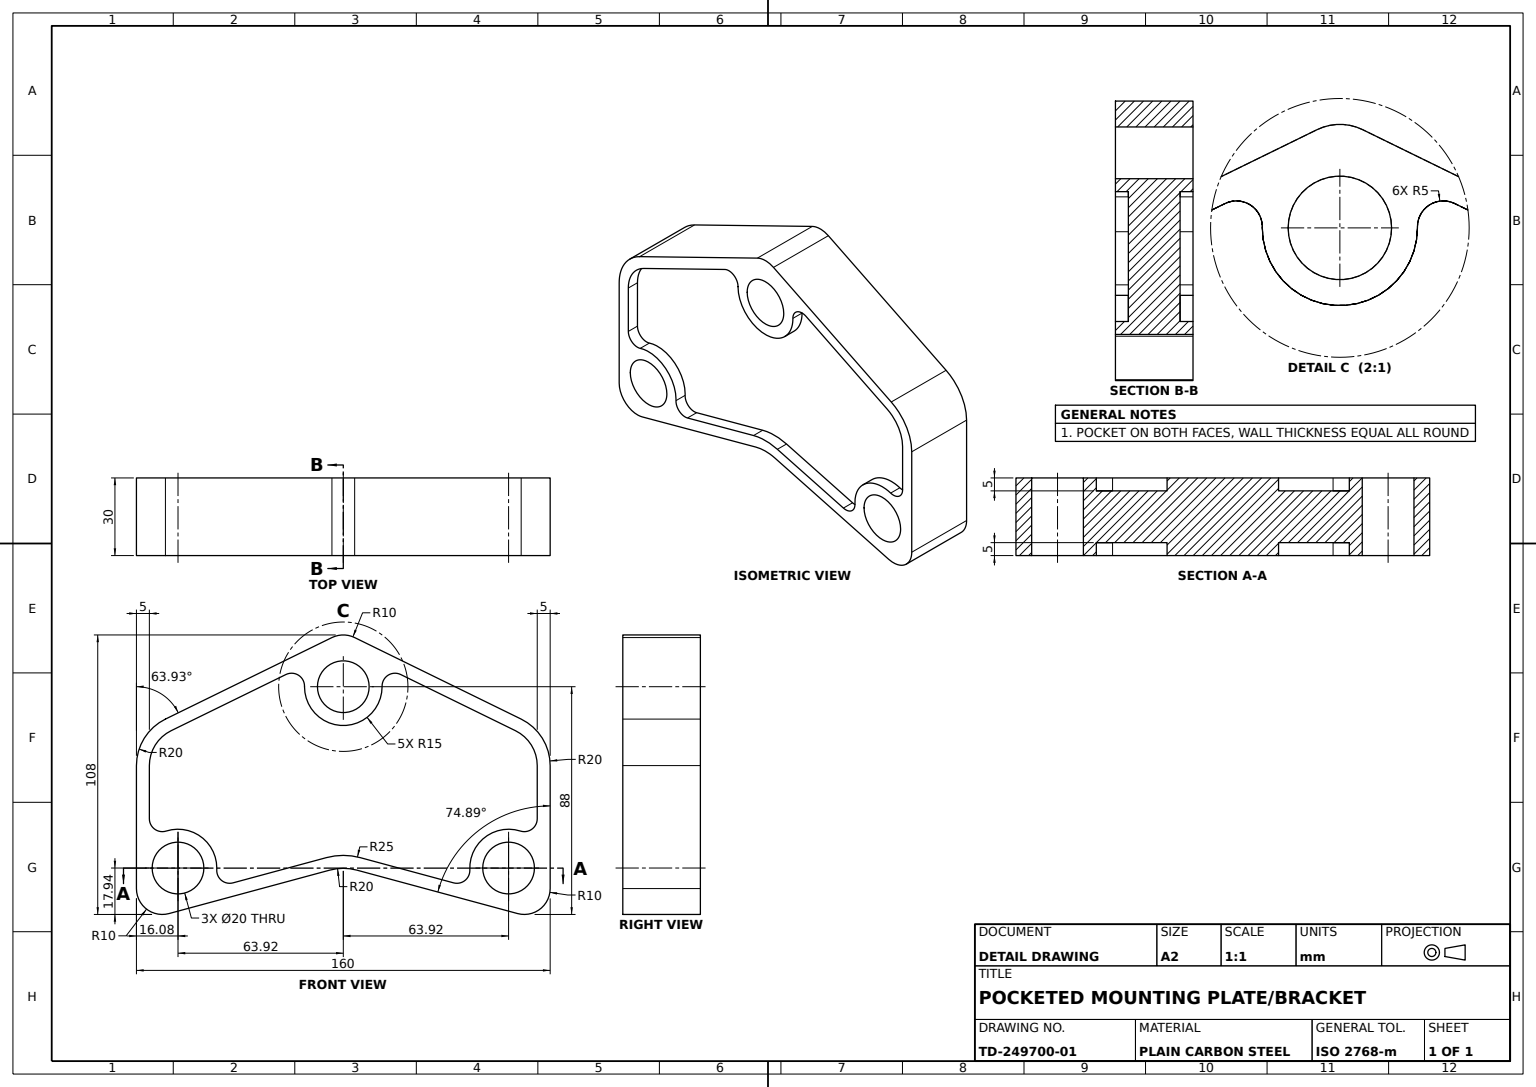
solid
v1 (-15,-10,15)
v2 (15,-10,15)
e1 v1 v2 CIRCLE(AX(P(0,-10,15),D(0,0,1),D(1,0,0)),15)
v3 (-15,-10,10)
e2 v3 v1 LINE
v4 (15,-10,10)
e3 v3 v4 CIRCLE(AX(P(0,-10,10),D(0,0,1),D(1,0,0)),15)
e4 v4 v2 LINE
face CYL(AX(P(0,-10,10),D(0,0,1),D(1,0,0)),15) [-e1 -e2 e3 e4]
v5 (-80,-40.481445,15)
v6 (-80,-88,15)
e5 v5 v6 LINE
v7 (-80,-40.481445,-15)
e6 v5 v7 LINE
v8 (-80,-88,-15)
e7 v7 v8 LINE
e8 v6 v8 LINE
face PLANE(AX(P(-80,-88,15),D(1,0,0),D(0,0,-1))) rev [-e5 e6 e7 -e8]
v9 (75,-61.007005,-15)
v10 (75,-40.481445,-15)
e9 v9 v10 LINE
v11 (75,-61.007005,-10)
e10 v11 v9 LINE
v12 (75,-40.481445,-10)
e11 v11 v12 LINE
e12 v12 v10 LINE
face PLANE(AX(P(75,-61.007005,-10),D(-1,0,0),D(0,-1,0))) [-e9 -e10 e11 e12]
v13 (-14.999113,-9.836864,-10)
v14 (-22.195826,-5.291032,-10)
e13 v13 v14 CIRCLE(AX(P(-19.998817,-9.782485,-10),D(0,0,1),D(1,0,0)),5)
v15 (-22.195826,-5.291032,-15)
e14 v14 v15 LINE
v16 (-14.999113,-9.836864,-15)
e15 v16 v15 CIRCLE(AX(P(-19.998817,-9.782485,-15),D(0,0,1),D(1,0,0)),5)
e16 v13 v16 LINE
face CYL(AX(P(-19.998817,-9.782485,-10),D(0,0,-1),D(-1,0,0)),5) rev [e13 e14 -e15 -e16]
v17 (-48.935435,-80.737052,10)
v18 (-42.636957,-85.789651,10)
e17 v17 v18 CIRCLE(AX(P(-43.940523,-80.96257,10),D(0,0,1),D(1,0,0)),5)
v19 (-48.935435,-80.737052,15)
e18 v17 v19 LINE
v20 (-42.636957,-85.789651,15)
e19 v19 v20 CIRCLE(AX(P(-43.940523,-80.96257,15),D(0,0,1),D(1,0,0)),5)
e20 v18 v20 LINE
face CYL(AX(P(-43.940523,-80.96257,10),D(0,0,1),D(1,0,0)),5) rev [-e17 e18 e19 -e20]
v21 (-15,-10,-10)
v22 (-15,-10,-15)
e21 v21 v22 LINE
e22 v13 v21 CIRCLE(AX(P(0,-10,-10),D(0,0,1),D(1,0,0)),15)
e23 v16 v22 CIRCLE(AX(P(0,-10,-15),D(0,0,1),D(1,0,0)),15)
face CYL(AX(P(0,-10,-10),D(0,0,-1),D(-1,0,0)),15) [-e21 -e22 e16 e23]
v23 (-4.394017,8.982907,15)
v24 (-4.394017,8.982907,-15)
e24 v23 v24 LINE
v25 (4.394017,8.982907,15)
e25 v25 v23 CIRCLE(AX(P(0,0,15),D(0,0,1),D(1,0,0)),10)
v26 (4.394017,8.982907,-15)
e26 v25 v26 LINE
e27 v26 v24 CIRCLE(AX(P(0,0,-15),D(0,0,1),D(1,0,0)),10)
face CYL(AX(P(0,0,15),D(0,0,-1),D(-1,0,0)),10) [-e24 -e25 e26 e27]
v27 (-48.920169,-80.0605,10)
v28 (-48.920169,-80.0605,15)
e28 v27 v28 LINE
v29 (-68.480042,-65.770379,10)
e29 v27 v29 CIRCLE(AX(P(-63.920169,-80.0605,10),D(0,0,1),D(1,0,0)),15)
v30 (-68.480042,-65.770379,15)
e30 v29 v30 LINE
e31 v28 v30 CIRCLE(AX(P(-63.920169,-80.0605,15),D(0,0,1),D(1,0,0)),15)
face CYL(AX(P(-63.920169,-80.0605,10),D(0,0,1),D(1,0,0)),15) [-e28 e29 e30 -e31]
v31 (-75,-40.481445,-10)
v32 (-75,-61.007005,-10)
e32 v31 v32 LINE
v33 (-75,-61.007005,-15)
e33 v32 v33 LINE
v34 (-75,-40.481445,-15)
e34 v34 v33 LINE
e35 v31 v34 LINE
face PLANE(AX(P(-75,-40.481445,-10),D(1,0,0),D(0,0,-1))) [e32 e33 -e34 -e35]
v35 (-75,-61.007005,15)
e36 v35 v30 CIRCLE(AX(P(-70,-61.007005,15),D(0,0,1),D(1,0,0)),5)
v36 (-75,-61.007005,10)
e37 v36 v29 CIRCLE(AX(P(-70,-61.007005,10),D(0,0,1),D(1,0,0)),5)
e38 v36 v35 LINE
face CYL(AX(P(-70,-61.007005,10),D(0,0,1),D(1,0,0)),5) rev [e36 -e30 -e37 e38]
v37 (48.935435,-80.737052,-10)
v38 (48.920169,-80.0605,-10)
e39 v37 v38 CIRCLE(AX(P(63.920169,-80.0605,-10),D(0,0,-1),D(-1,0,0)),15)
v39 (42.636957,-85.789651,-10)
e40 v37 v39 CIRCLE(AX(P(43.940523,-80.96257,-10),D(0,0,-1),D(-1,0,0)),5)
v40 (6.51783,-76.035586,-10)
e41 v40 v39 LINE
v41 (-6.51783,-76.035586,-10)
e42 v40 v41 CIRCLE(AX(P(0,-100.170994,-10),D(0,0,1),D(1,0,0)),25)
v42 (-42.636957,-85.789651,-10)
e43 v42 v41 LINE
v43 (-48.940523,-80.96257,-10)
e44 v43 v42 CIRCLE(AX(P(-43.940523,-80.96257,-10),D(0,0,1),D(1,0,0)),5)
v44 (-48.935435,-80.737052,-10)
e45 v44 v43 CIRCLE(AX(P(-43.940523,-80.96257,-10),D(0,0,1),D(1,0,0)),5)
v45 (-68.480042,-65.770379,-10)
e46 v44 v45 CIRCLE(AX(P(-63.920169,-80.0605,-10),D(0,0,1),D(1,0,0)),15)
e47 v32 v45 CIRCLE(AX(P(-70,-61.007005,-10),D(0,0,1),D(1,0,0)),5)
v46 (-66.591026,-27.007085,-10)
e48 v46 v31 CIRCLE(AX(P(-60,-40.481445,-10),D(0,0,1),D(1,0,0)),15)
e49 v14 v46 LINE
v47 (15,-10,-10)
e50 v21 v47 CIRCLE(AX(P(0,-10,-10),D(0,0,1),D(1,0,0)),15)
v48 (14.999113,-9.836864,-10)
e51 v47 v48 CIRCLE(AX(P(0,-10,-10),D(0,0,1),D(1,0,0)),15)
v49 (14.998817,-9.782485,-10)
e52 v48 v49 CIRCLE(AX(P(19.998817,-9.782485,-10),D(0,0,-1),D(-1,0,0)),5)
v50 (22.195826,-5.291032,-10)
e53 v49 v50 CIRCLE(AX(P(19.998817,-9.782485,-10),D(0,0,-1),D(-1,0,0)),5)
v51 (66.591026,-27.007085,-10)
e54 v51 v50 LINE
e55 v12 v51 CIRCLE(AX(P(60,-40.481445,-10),D(0,0,1),D(1,0,0)),15)
v52 (68.480042,-65.770379,-10)
e56 v11 v52 CIRCLE(AX(P(70,-61.007005,-10),D(0,0,-1),D(-1,0,0)),5)
e57 v38 v52 CIRCLE(AX(P(63.920169,-80.0605,-10),D(0,0,-1),D(-1,0,0)),15)
face PLANE(AX(P(70,-61.007005,-10),D(0,0,1),D(-1,0,0))) rev [-e39 e40 -e41 e42 -e43 -e44 -e45 e46 -e47 -e32 -e48 -e49 -e13 e22 e50 e51 e52 e53 -e54 -e55 -e11 e56 -e57]
v53 (14.998817,-9.782485,-15)
e58 v49 v53 LINE
v54 (22.195826,-5.291032,-15)
e59 v53 v54 CIRCLE(AX(P(19.998817,-9.782485,-15),D(0,0,-1),D(-1,0,0)),5)
e60 v50 v54 LINE
face CYL(AX(P(19.998817,-9.782485,-10),D(0,0,-1),D(-1,0,0)),5) rev [e58 e59 -e60 -e53]
v55 (42.636957,-85.789651,10)
v56 (42.636957,-85.789651,15)
e61 v55 v56 LINE
v57 (6.51783,-76.035586,10)
e62 v57 v55 LINE
v58 (6.51783,-76.035586,15)
e63 v57 v58 LINE
e64 v58 v56 LINE
face PLANE(AX(P(6.51783,-76.035586,10),D(-0.260713207,-0.965416296,0),D(0.965416296,-0.260713207,0))) rev [-e61 -e62 e63 e64]
v59 (-53.920169,-80.0605,15)
v60 (-73.920169,-80.0605,15)
e65 v59 v60 CIRCLE(AX(P(-63.920169,-80.0605,15),D(0,0,1),D(1,0,0)),10)
e66 v60 v59 CIRCLE(AX(P(-63.920169,-80.0605,15),D(0,0,1),D(1,0,0)),10)
v61 (-14.998817,-9.782485,15)
v62 (-22.195826,-5.291032,15)
e67 v61 v62 CIRCLE(AX(P(-19.998817,-9.782485,15),D(0,0,1),D(1,0,0)),5)
v63 (-14.999113,-9.836864,15)
e68 v63 v61 CIRCLE(AX(P(-19.998817,-9.782485,15),D(0,0,1),D(1,0,0)),5)
e69 v63 v1 CIRCLE(AX(P(0,-10,15),D(0,0,1),D(1,0,0)),15)
v64 (14.999113,-9.836864,15)
e70 v2 v64 CIRCLE(AX(P(0,-10,15),D(0,0,1),D(1,0,0)),15)
v65 (22.195826,-5.291032,15)
e71 v64 v65 CIRCLE(AX(P(19.998817,-9.782485,15),D(0,0,-1),D(-1,0,0)),5)
v66 (66.591026,-27.007085,15)
e72 v66 v65 LINE
v67 (75,-40.481445,15)
e73 v67 v66 CIRCLE(AX(P(60,-40.481445,15),D(0,0,1),D(1,0,0)),15)
v68 (75,-61.007005,15)
e74 v68 v67 LINE
v69 (68.480042,-65.770379,15)
e75 v68 v69 CIRCLE(AX(P(70,-61.007005,15),D(0,0,-1),D(-1,0,0)),5)
v70 (48.935435,-80.737052,15)
e76 v70 v69 CIRCLE(AX(P(63.920169,-80.0605,15),D(0,0,-1),D(-1,0,0)),15)
v71 (48.940523,-80.96257,15)
e77 v70 v71 CIRCLE(AX(P(43.940523,-80.96257,15),D(0,0,-1),D(-1,0,0)),5)
e78 v71 v56 CIRCLE(AX(P(43.940523,-80.96257,15),D(0,0,-1),D(-1,0,0)),5)
v72 (-6.51783,-76.035586,15)
e79 v58 v72 CIRCLE(AX(P(0,-100.170994,15),D(0,0,1),D(1,0,0)),25)
e80 v20 v72 LINE
e81 v19 v28 CIRCLE(AX(P(-63.920169,-80.0605,15),D(0,0,1),D(1,0,0)),15)
v73 (-75,-40.481445,15)
e82 v73 v35 LINE
v74 (-66.591026,-27.007085,15)
e83 v74 v73 CIRCLE(AX(P(-60,-40.481445,15),D(0,0,1),D(1,0,0)),15)
e84 v62 v74 LINE
v75 (68.788035,-22.515632,15)
e85 v75 v25 LINE
v76 (-68.788035,-22.515632,15)
e86 v23 v76 LINE
e87 v76 v5 CIRCLE(AX(P(-60,-40.481445,15),D(0,0,1),D(-1,0,0)),20)
v77 (-67.392868,-97.654163,15)
e88 v6 v77 CIRCLE(AX(P(-70,-88,15),D(0,0,1),D(1,0,0)),10)
v78 (-5.214264,-80.862668,15)
e89 v77 v78 LINE
v79 (5.214264,-80.862668,15)
e90 v78 v79 CIRCLE(AX(P(0,-100.170994,15),D(0,0,-1),D(-1,0,0)),20)
v80 (67.392868,-97.654163,15)
e91 v79 v80 LINE
v81 (80,-88,15)
e92 v80 v81 CIRCLE(AX(P(70,-88,15),D(0,0,1),D(1,0,0)),10)
v82 (80,-40.481445,15)
e93 v81 v82 LINE
e94 v82 v75 CIRCLE(AX(P(60,-40.481445,15),D(0,0,1),D(1,0,0)),20)
v83 (53.920169,-80.0605,15)
v84 (73.920169,-80.0605,15)
e95 v83 v84 CIRCLE(AX(P(63.920169,-80.0605,15),D(0,0,1),D(1,0,0)),10)
e96 v84 v83 CIRCLE(AX(P(63.920169,-80.0605,15),D(0,0,1),D(1,0,0)),10)
v85 (-10,-10,15)
v86 (10,-10,15)
e97 v85 v86 CIRCLE(AX(P(0,-10,15),D(0,0,1),D(1,0,0)),10)
e98 v86 v85 CIRCLE(AX(P(0,-10,15),D(0,0,1),D(1,0,0)),10)
face PLANE(AX(P(-60,-40.481445,15),D(0,0,-1),D(-1,0,0))) rev [-e65 -e66] [-e67 -e68 e69 e1 e70 e71 -e72 -e73 -e74 e75 -e76 e77 e78 -e64 e79 -e80 -e19 e81 e31 -e36 -e82 -e83 -e84] [e85 e25 e86 e87 e5 e88 e89 e90 e91 e92 e93 e94] [-e95 -e96] [-e97 -e98]
v87 (-48.935435,-80.737052,-15)
e99 v44 v87 LINE
v88 (-48.940523,-80.96257,-15)
e100 v43 v88 LINE
e101 v87 v88 CIRCLE(AX(P(-43.940523,-80.96257,-15),D(0,0,1),D(1,0,0)),5)
face CYL(AX(P(-43.940523,-80.96257,-10),D(0,0,-1),D(-1,0,0)),5) rev [-e99 e45 e100 -e101]
v89 (-68.788035,-22.515632,-15)
e102 v89 v7 CIRCLE(AX(P(-60,-40.481445,-15),D(0,0,1),D(-1,0,0)),20)
e103 v76 v89 LINE
face CYL(AX(P(-60,-40.481445,15),D(0,0,-1),D(-1,0,0)),20) [e102 -e6 -e87 e103]
v90 (48.935435,-80.737052,10)
v91 (48.940523,-80.96257,10)
e104 v90 v91 CIRCLE(AX(P(43.940523,-80.96257,10),D(0,0,-1),D(-1,0,0)),5)
e105 v91 v71 LINE
e106 v90 v70 LINE
face CYL(AX(P(43.940523,-80.96257,10),D(0,0,1),D(1,0,0)),5) rev [e104 e105 -e77 -e106]
v92 (48.920169,-80.0605,-15)
e107 v38 v92 LINE
v93 (68.480042,-65.770379,-15)
e108 v52 v93 LINE
e109 v92 v93 CIRCLE(AX(P(63.920169,-80.0605,-15),D(0,0,-1),D(-1,0,0)),15)
face CYL(AX(P(63.920169,-80.0605,-10),D(0,0,-1),D(-1,0,0)),15) [-e107 e57 e108 -e109]
v94 (-53.920169,-80.0605,-15)
v95 (-73.920169,-80.0605,-15)
e110 v94 v95 CIRCLE(AX(P(-63.920169,-80.0605,-15),D(0,0,1),D(1,0,0)),10)
e111 v95 v94 CIRCLE(AX(P(-63.920169,-80.0605,-15),D(0,0,1),D(1,0,0)),10)
v96 (10,-10,-15)
v97 (-10,-10,-15)
e112 v96 v97 CIRCLE(AX(P(0,-10,-15),D(0,0,1),D(1,0,0)),10)
e113 v97 v96 CIRCLE(AX(P(0,-10,-15),D(0,0,1),D(1,0,0)),10)
v98 (53.920169,-80.0605,-15)
v99 (73.920169,-80.0605,-15)
e114 v98 v99 CIRCLE(AX(P(63.920169,-80.0605,-15),D(0,0,1),D(1,0,0)),10)
e115 v99 v98 CIRCLE(AX(P(63.920169,-80.0605,-15),D(0,0,1),D(1,0,0)),10)
v100 (80,-88,-15)
v101 (80,-40.481445,-15)
e116 v100 v101 LINE
v102 (67.392868,-97.654163,-15)
e117 v102 v100 CIRCLE(AX(P(70,-88,-15),D(0,0,1),D(1,0,0)),10)
v103 (5.214264,-80.862668,-15)
e118 v103 v102 LINE
v104 (-5.214264,-80.862668,-15)
e119 v104 v103 CIRCLE(AX(P(0,-100.170994,-15),D(0,0,-1),D(-1,0,0)),20)
v105 (-67.392868,-97.654163,-15)
e120 v105 v104 LINE
e121 v8 v105 CIRCLE(AX(P(-70,-88,-15),D(0,0,1),D(1,0,0)),10)
e122 v24 v89 LINE
v106 (68.788035,-22.515632,-15)
e123 v106 v26 LINE
e124 v101 v106 CIRCLE(AX(P(60,-40.481445,-15),D(0,0,1),D(1,0,0)),20)
v107 (66.591026,-27.007085,-15)
e125 v10 v107 CIRCLE(AX(P(60,-40.481445,-15),D(0,0,1),D(1,0,0)),15)
e126 v107 v54 LINE
v108 (14.999113,-9.836864,-15)
e127 v108 v53 CIRCLE(AX(P(19.998817,-9.782485,-15),D(0,0,-1),D(-1,0,0)),5)
v109 (15,-10,-15)
e128 v109 v108 CIRCLE(AX(P(0,-10,-15),D(0,0,1),D(1,0,0)),15)
e129 v22 v109 CIRCLE(AX(P(0,-10,-15),D(0,0,1),D(1,0,0)),15)
v110 (-66.591026,-27.007085,-15)
e130 v15 v110 LINE
e131 v110 v34 CIRCLE(AX(P(-60,-40.481445,-15),D(0,0,1),D(1,0,0)),15)
v111 (-68.480042,-65.770379,-15)
e132 v33 v111 CIRCLE(AX(P(-70,-61.007005,-15),D(0,0,1),D(1,0,0)),5)
e133 v87 v111 CIRCLE(AX(P(-63.920169,-80.0605,-15),D(0,0,1),D(1,0,0)),15)
v112 (-42.636957,-85.789651,-15)
e134 v88 v112 CIRCLE(AX(P(-43.940523,-80.96257,-15),D(0,0,1),D(1,0,0)),5)
v113 (-6.51783,-76.035586,-15)
e135 v112 v113 LINE
v114 (6.51783,-76.035586,-15)
e136 v114 v113 CIRCLE(AX(P(0,-100.170994,-15),D(0,0,1),D(1,0,0)),25)
v115 (42.636957,-85.789651,-15)
e137 v114 v115 LINE
v116 (48.935435,-80.737052,-15)
e138 v116 v115 CIRCLE(AX(P(43.940523,-80.96257,-15),D(0,0,-1),D(-1,0,0)),5)
e139 v116 v92 CIRCLE(AX(P(63.920169,-80.0605,-15),D(0,0,-1),D(-1,0,0)),15)
e140 v9 v93 CIRCLE(AX(P(70,-61.007005,-15),D(0,0,-1),D(-1,0,0)),5)
face PLANE(AX(P(-60,-40.481445,-15),D(0,0,-1),D(-1,0,0))) [e110 e111] [e112 e113] [e114 e115] [-e116 -e117 -e118 -e119 -e120 -e121 -e7 -e102 -e122 -e27 -e123 -e124] [e125 e126 -e59 -e127 -e128 -e129 -e23 e15 e130 e131 e34 e132 -e133 e101 e134 e135 -e136 e137 -e138 e139 e109 -e140 e9]
v117 (66.591026,-27.007085,10)
v118 (22.195826,-5.291032,10)
e141 v117 v118 LINE
e142 v117 v66 LINE
e143 v118 v65 LINE
face PLANE(AX(P(66.591026,-27.007085,10),D(0.439401732,0.898290664,0),D(-0.898290664,0.439401732,0))) rev [-e141 e142 e72 -e143]
e144 v51 v107 LINE
face PLANE(AX(P(66.591026,-27.007085,-10),D(-0.439401732,-0.898290664,0),D(0.898290664,-0.439401732,0))) [e54 e60 -e126 -e144]
v119 (-14.998817,-9.782485,10)
v120 (-22.195826,-5.291032,10)
e145 v119 v120 CIRCLE(AX(P(-19.998817,-9.782485,10),D(0,0,1),D(1,0,0)),5)
e146 v119 v61 LINE
e147 v120 v62 LINE
face CYL(AX(P(-19.998817,-9.782485,10),D(0,0,1),D(1,0,0)),5) rev [-e145 e146 e67 -e147]
e148 v39 v115 LINE
e149 v37 v116 LINE
face CYL(AX(P(43.940523,-80.96257,-10),D(0,0,-1),D(-1,0,0)),5) rev [e138 -e148 -e40 e149]
e150 v96 v86 LINE
e151 v97 v85 LINE
face CYL(AX(P(0,-10,-15),D(0,0,1),D(1,0,0)),10) rev [-e150 -e113 e151 e97]
e152 v46 v110 LINE
face CYL(AX(P(-60,-40.481445,-10),D(0,0,-1),D(-1,0,0)),15) rev [-e152 e48 e35 -e131]
v121 (-6.51783,-76.035586,10)
e153 v121 v72 LINE
e154 v18 v121 LINE
face PLANE(AX(P(-42.636957,-85.789651,10),D(0.260713207,-0.965416296,0),D(0.965416296,0.260713207,0))) rev [e20 e80 -e153 -e154]
e155 v75 v106 LINE
face PLANE(AX(P(68.788035,-22.515632,15),D(-0.439401732,-0.898290664,0),D(0.898290664,-0.439401732,0))) rev [-e85 e155 e123 -e26]
e156 v17 v27 CIRCLE(AX(P(-63.920169,-80.0605,10),D(0,0,1),D(1,0,0)),15)
face CYL(AX(P(-63.920169,-80.0605,10),D(0,0,1),D(1,0,0)),15) [e28 -e81 -e18 e156]
v122 (75,-40.481445,10)
e157 v122 v117 CIRCLE(AX(P(60,-40.481445,10),D(0,0,1),D(1,0,0)),15)
e158 v122 v67 LINE
face CYL(AX(P(60,-40.481445,10),D(0,0,1),D(1,0,0)),15) rev [-e157 e158 e73 -e142]
v123 (75,-61.007005,10)
e159 v123 v122 LINE
e160 v123 v68 LINE
face PLANE(AX(P(75,-61.007005,10),D(1,0,0),D(0,1,0))) rev [e74 -e158 -e159 e160]
e161 v81 v100 LINE
e162 v80 v102 LINE
face CYL(AX(P(70,-88,15),D(0,0,-1),D(-1,0,0)),10) [e117 -e161 -e92 e162]
e163 v47 v109 LINE
e164 v48 v108 LINE
face CYL(AX(P(0,-10,-10),D(0,0,-1),D(-1,0,0)),15) [e163 e128 -e164 -e51]
face CYL(AX(P(19.998817,-9.782485,-10),D(0,0,-1),D(-1,0,0)),5) rev [e127 -e58 -e52 e164]
v124 (-14.999113,-9.836864,10)
e165 v124 v119 CIRCLE(AX(P(-19.998817,-9.782485,10),D(0,0,1),D(1,0,0)),5)
e166 v124 v63 LINE
face CYL(AX(P(-19.998817,-9.782485,10),D(0,0,1),D(1,0,0)),5) rev [e68 -e146 -e165 e166]
e167 v42 v112 LINE
face CYL(AX(P(-43.940523,-80.96257,-10),D(0,0,-1),D(-1,0,0)),5) rev [-e100 e44 e167 -e134]
face CYL(AX(P(0,-10,-10),D(0,0,-1),D(-1,0,0)),15) [-e50 e21 e129 -e163]
face PLANE(AX(P(-22.195826,-5.291032,-10),D(0.439401732,-0.898290664,0),D(0.898290664,0.439401732,0))) [-e14 e49 e152 -e130]
v125 (68.480042,-65.770379,10)
e168 v90 v125 CIRCLE(AX(P(63.920169,-80.0605,10),D(0,0,-1),D(-1,0,0)),15)
e169 v125 v69 LINE
face CYL(AX(P(63.920169,-80.0605,10),D(0,0,1),D(1,0,0)),15) [-e168 e106 e76 -e169]
face CYL(AX(P(70,-61.007005,-10),D(0,0,-1),D(-1,0,0)),5) rev [-e108 -e56 e10 e140]
v126 (-66.591026,-27.007085,10)
e170 v126 v74 LINE
e171 v120 v126 LINE
face PLANE(AX(P(-22.195826,-5.291032,10),D(-0.439401732,0.898290664,0),D(-0.898290664,-0.439401732,0))) rev [e84 -e170 -e171 e147]
e172 v94 v59 LINE
e173 v95 v60 LINE
face CYL(AX(P(-63.920169,-80.0605,-15),D(0,0,1),D(1,0,0)),10) rev [-e110 e172 e65 -e173]
face CYL(AX(P(60,-40.481445,-10),D(0,0,-1),D(-1,0,0)),15) rev [-e12 e55 e144 -e125]
e174 v41 v113 LINE
face PLANE(AX(P(-42.636957,-85.789651,-10),D(-0.260713207,0.965416296,0),D(-0.965416296,-0.260713207,0))) [e174 -e135 -e167 e43]
e175 v82 v101 LINE
face CYL(AX(P(60,-40.481445,15),D(0,0,-1),D(-1,0,0)),20) [e124 -e155 -e94 e175]
e176 v45 v111 LINE
face CYL(AX(P(-70,-61.007005,-10),D(0,0,-1),D(-1,0,0)),5) rev [e47 e176 -e132 -e33]
e177 v123 v125 CIRCLE(AX(P(70,-61.007005,10),D(0,0,-1),D(-1,0,0)),5)
face CYL(AX(P(70,-61.007005,10),D(0,0,1),D(1,0,0)),5) rev [e177 e169 -e75 -e160]
v127 (14.999113,-9.836864,10)
e178 v4 v127 CIRCLE(AX(P(0,-10,10),D(0,0,1),D(1,0,0)),15)
e179 v127 v64 LINE
face CYL(AX(P(0,-10,10),D(0,0,1),D(1,0,0)),15) [-e70 -e4 e178 e179]
face CYL(AX(P(-63.920169,-80.0605,-10),D(0,0,-1),D(-1,0,0)),15) [e133 -e176 -e46 e99]
v128 (-75,-40.481445,10)
e180 v128 v36 LINE
e181 v128 v73 LINE
face PLANE(AX(P(-75,-40.481445,10),D(-1,0,0),D(0,0,1))) rev [-e38 -e180 e181 e82]
e182 v127 v118 CIRCLE(AX(P(19.998817,-9.782485,10),D(0,0,-1),D(-1,0,0)),5)
face CYL(AX(P(19.998817,-9.782485,10),D(0,0,1),D(1,0,0)),5) rev [e182 e143 -e71 -e179]
face CYL(AX(P(63.920169,-80.0605,-10),D(0,0,-1),D(-1,0,0)),15) [-e139 -e149 e39 e107]
e183 v77 v105 LINE
face CYL(AX(P(-70,-88,15),D(0,0,-1),D(-1,0,0)),10) [-e88 e8 e121 -e183]
e184 v98 v83 LINE
e185 v99 v84 LINE
face CYL(AX(P(63.920169,-80.0605,-15),D(0,0,1),D(1,0,0)),10) rev [e96 -e184 -e115 e185]
face PLANE(AX(P(-68.788035,-22.515632,15),D(0.439401732,-0.898290664,0),D(0.898290664,0.439401732,0))) rev [-e103 -e86 e24 e122]
e186 v78 v104 LINE
face PLANE(AX(P(-67.392868,-97.654163,15),D(-0.260713207,0.965416296,0),D(-0.965416296,-0.260713207,0))) rev [-e186 -e89 e183 e120]
e187 v40 v114 LINE
face PLANE(AX(P(6.51783,-76.035586,-10),D(0.260713207,0.965416296,0),D(-0.965416296,0.260713207,0))) [-e137 -e187 e41 e148]
face PLANE(AX(P(80,-88,15),D(-1,0,0),D(0,0,1))) rev [e161 e116 -e175 -e93]
e188 v126 v128 CIRCLE(AX(P(-60,-40.481445,10),D(0,0,1),D(1,0,0)),15)
e189 v57 v121 CIRCLE(AX(P(0,-100.170994,10),D(0,0,1),D(1,0,0)),25)
e190 v91 v55 CIRCLE(AX(P(43.940523,-80.96257,10),D(0,0,-1),D(-1,0,0)),5)
e191 v124 v3 CIRCLE(AX(P(0,-10,10),D(0,0,1),D(1,0,0)),15)
face PLANE(AX(P(70,-61.007005,10),D(0,0,-1),D(-1,0,0))) rev [e188 e180 e37 -e29 -e156 e17 e154 -e189 e62 -e190 -e104 e168 -e177 e159 e157 e141 -e182 -e178 -e3 -e191 e165 e145 e171]
e192 v79 v103 LINE
face PLANE(AX(P(5.214264,-80.862668,15),D(0.260713207,0.965416296,0),D(-0.965416296,0.260713207,0))) rev [e118 -e162 -e91 e192]
face CYL(AX(P(63.920169,-80.0605,-15),D(0,0,1),D(1,0,0)),10) rev [-e114 e184 e95 -e185]
face CYL(AX(P(43.940523,-80.96257,10),D(0,0,1),D(1,0,0)),5) rev [e190 e61 -e78 -e105]
face CYL(AX(P(-60,-40.481445,10),D(0,0,1),D(1,0,0)),15) rev [e170 e83 -e181 -e188]
face CYL(AX(P(0,-10,-15),D(0,0,1),D(1,0,0)),10) rev [-e112 e150 e98 -e151]
face CYL(AX(P(-63.920169,-80.0605,-15),D(0,0,1),D(1,0,0)),10) rev [-e172 -e111 e173 e66]
face CYL(AX(P(0,-100.170994,10),D(0,0,1),D(1,0,0)),25) [e153 -e79 -e63 e189]
face CYL(AX(P(0,-100.170994,-10),D(0,0,-1),D(-1,0,0)),25) [-e174 -e42 e187 e136]
face CYL(AX(P(0,-100.170994,15),D(0,0,-1),D(-1,0,0)),20) rev [-e192 -e90 e186 e119]
face CYL(AX(P(0,-10,10),D(0,0,1),D(1,0,0)),15) [e2 -e69 -e166 e191]
